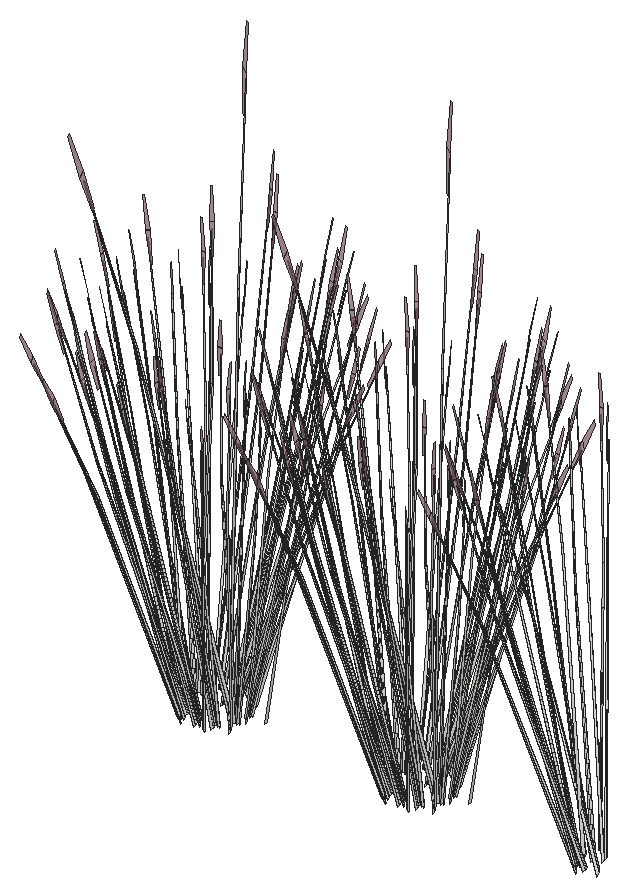
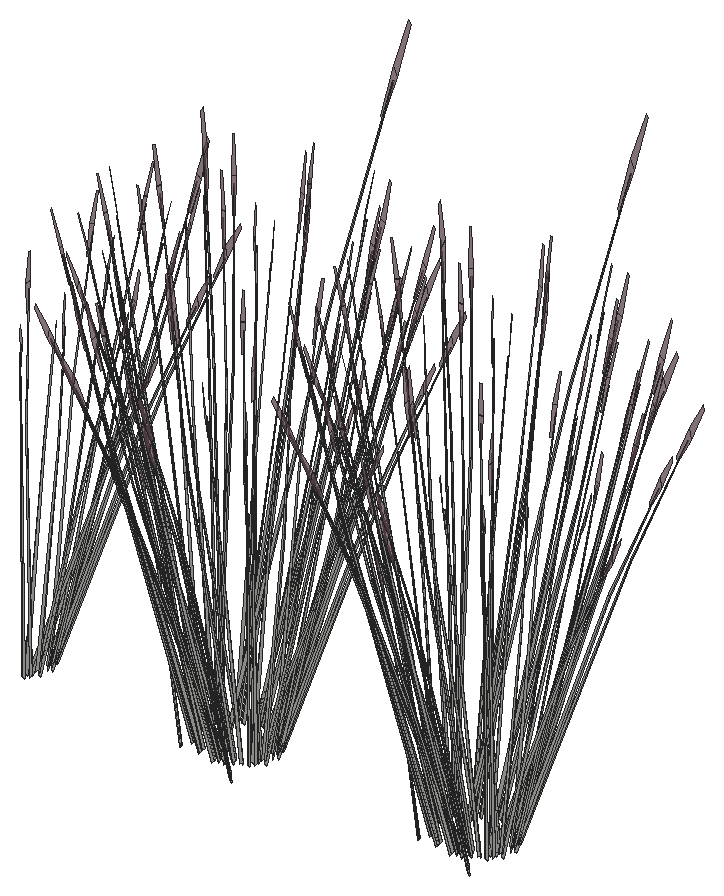
# SketchUp Ruby script. Lengths in inches.
U = 1.inch
M = Sketchup.active_model
def pt(a) = Geom::Point3d.new(a.map { |v| v * U })
def face(e, loops, mat)
  f = e.add_face(loops[0].map { |a| pt(a) })
  loops[1..].each { |l| e.add_face(l.map { |a| pt(a) }).erase! }
  f.material = f.back_material = mat if mat
  f
end
# faces: each face lists its corners as indices into pts; further lists are holes
def faces(e, pts, list, mat = nil) = list.each { |f| face(e, (f[0].is_a?(Array) ? f : [f]).map { |l| l.map { |i| pts[i] } }, mat) }
# xy, xz, yz: faces in a plane at the given z, y or x. An outline is a flat list of corners, or four numbers for a rectangle; further outlines are holes
def ring(l) = l.size == 4 ? [[l[0], l[1]], [l[2], l[1]], [l[2], l[3]], [l[0], l[3]]] : l.each_slice(2).to_a
def flat(e, list, mat, &to3) = list.each { |f| face(e, (f[0].is_a?(Array) ? f : [f]).map { |l| ring(l).map { |u, v| to3.(u, v) } }, mat) }
def xy(e, z, list, mat = nil) = flat(e, list, mat) { |x, y| [x, y, z] }
def xz(e, y, list, mat = nil) = flat(e, list, mat) { |x, z| [x, y, z] }
def yz(e, x, list, mat = nil) = flat(e, list, mat) { |y, z| [x, y, z] }
def lines(e, pts, list) = list.each { |a, b| e.add_line(pt(pts[a]), pt(pts[b])) }
# prism: a flat outline (further loops are holes) pulled along v
def prism(e, loops, v, mat = nil)
  f = face(e, loops, mat); d = Geom::Vector3d.new(v.map { |x| x * U })
  f.pushpull(f.normal.samedirection?(d) ? d.length : -d.length)
end
def box(e, o, s, mat = nil) = prism(e, [[o, [o[0] + s[0], o[1], o[2]], [o[0] + s[0], o[1] + s[1], o[2]], [o[0], o[1] + s[1], o[2]]]], [0, 0, s[2]], mat)
def at(x, y, z, deg = 0) = Geom::Transformation.translation(pt([x, y, z])) * Geom::Transformation.rotation(ORIGIN, Z_AXIS, deg.degrees)
def axes(o, x, y, z) = Geom::Transformation.new([*x, 0, *y, 0, *z, 0, *pt(o).to_a, 1])
def part(name) = M.definitions.add(name)
# library, detail: a bought-in or finely detailed component or shape, given as its bounding box
def library(name, o, s) = part(name).tap { |d| box(d.entities, o, s) }
def detail(e, o, s) = box(e.add_group.entities, o, s)
def put(e, d, t, mat = nil) = e.add_instance(d, t).tap { |i| i.material = mat if mat }
def group(e, t, mat = nil) = e.add_group.tap { |g| g.transformation = t; g.material = mat if mat }.entities
root = M.entities
M.materials.add("LightPink_Translucent").color = [144, 107, 117]
M.materials["LightPink_Translucent"].alpha = 0.75
c1 = part("blade")
p = [[2.15,0.21,22],[0,0.17,0],[0.09,0.45,0],[2.18,0.31,22],[2.29,0.31,22],[0.38,0.45,0],
  [2.48,0.24,33],[2.49,0.24,33],[2.48,0.22,33]]
faces(c1.entities,p,[[0,1,2,3],[4,5,2,3],[6,3,4,7],[8,0,3,6]])
c2 = part("seeds")
p = [[0.3,-0.1,1.38],[-0.01,-0.03,1.59],[-0.01,-0.03,0.03],[0.14,-0.07,-0.07],[0.29,-0.03,3],[0.15,0.01,3.11]]
faces(c2.entities,p,[[0,1,2,3],[1,0,4,5]],"LightPink_Translucent")
c3 = part("blade with seeds")
put(c3.entities,c1,at(0,0,0))
put(c3.entities,c2,axes([2.4,0.25,30.99],[1.5799,-0.05474,1.17369],[-0.12525,1.92788,0.29478],[-0.07173,-0.02425,1.56792]))
put(root,c3,axes([283.23,56.33,267.61],[0.21212,-0.01231,1.59586],[-0.14072,0.53355,0.12904],[-0.3023,-0.033,0.68222]))
put(root,c3,axes([283.32,57.27,267.61],[0.17745,-0.11497,1.59586],[0.14939,0.53127,0.12904],[-0.27857,0.12007,0.68222]))
put(root,c3,axes([284.33,56.71,267.11],[0.14537,-0.07863,1.64882],[0.05013,0.549,0.12904],[-0.31487,0.07285,0.5893]))
put(root,c3,axes([283.86,55.83,268.64],[-0.51122,-0.01309,-0.66157],[0.03434,-0.5511,0.07984],[-0.21658,-0.05816,0.93586]))
put(root,c3,axes([283.04,56.79,268.22],[-0.42502,-0.15163,-0.32977],[0.12396,-0.44238,0.42575],[-0.17112,0.04056,0.81462]))
put(root,c3,axes([283.63,55.47,267.61],[0.18996,0.09365,1.59586],[-0.39312,0.39287,0.12904],[-0.24502,-0.17723,0.68222]))
put(root,c3,axes([283.33,57.01,268.36],[-0.13855,0.49442,-0.47583],[-0.47502,-0.16947,-0.36857],[-0.19125,0.04534,0.91046]))
put(root,c3,axes([283.69,55.94,268.36],[-0.37135,0.36005,-0.47583],[-0.32522,-0.38035,-0.36857],[-0.18868,-0.05478,0.91046]))
put(root,c3,axes([283.31,56.59,268.6875],[0.25732,0.49218,-0.11324],[-0.45669,0.24187,-0.62851],[-0.19245,0.06494,0.95501]))
put(root,c3,axes([283.89,55.57,268.6875],[-0.02738,0.55277,-0.11324],[-0.51847,-0.01511,-0.62851],[-0.19968,-0.0384,0.95501]))
put(root,c3,axes([283.55,55.6,268.22],[-0.29098,-0.34031,-0.32977],[0.33226,-0.32215,0.42575],[-0.16881,-0.04902,0.81462]))
put(root,c3,axes([283.96,57.625,267.61],[0.12773,-0.16701,1.59586],[0.32252,0.4508,0.12904],[-0.22121,0.20529,0.68222]))
put(root,c3,axes([283.2,58.0625,268.22],[-0.44516,0.07768,-0.32977],[-0.11755,-0.44407,0.42575],[-0.12757,0.11927,0.81462]))
put(root,c3,axes([283.87,58.04,267.61],[0.09522,-0.18683,1.59586],[0.39947,0.38663,0.12904],[-0.18021,0.24097,0.68222]))
put(root,c3,axes([283.5625,58.11,268.36],[0.13138,0.49631,-0.47583],[-0.49754,0.08682,-0.36857],[-0.14258,0.13331,0.91046]))
put(root,c3,axes([284.75,55.18,268.64],[-0.43608,-0.26272,-0.66157],[0.30991,-0.46038,0.07984],[-0.158,-0.15687,0.93586]))
put(root,c3,axes([284.55,55.2,268.36],[-0.50465,0.12921,-0.47583],[-0.08828,-0.48932,-0.36857],[-0.13555,-0.14022,0.91046]))
put(root,c3,axes([283.33,57.76,268.6875],[0.47307,0.29971,-0.11324],[-0.27254,0.43404,-0.62851],[-0.13365,0.15087,0.95501]))
put(root,c3,axes([284.41,54.93,267.61],[0.1169,0.17452,1.59586],[-0.54019,0.14692,0.12904],[-0.12209,-0.27397,0.68222]))
put(root,c3,axes([284.6,54.83,268.22],[-0.07899,-0.43781,-0.32977],[0.45153,-0.11561,0.42575],[-0.12128,-0.12546,0.81462]))
put(root,c3,axes([283.98,59.09,268.22],[-0.34603,0.28618,-0.32977],[-0.32756,-0.32677,0.42575],[-0.04984,0.16603,0.81462]))
put(root,c3,axes([285.79,58.15,267.1],[0.44194,0.21918,1.40854],[-0.43295,0.47219,0.557],[-0.19393,-0.27986,1.18082]))
put(root,c3,axes([284.21,58.79,268.97],[-0.01331,0.50278,-0.73435],[-0.56035,-0.03377,0.08862],[-0.05914,0.213,1.03881]))
put(root,c3,axes([284.02,59.5,267.13],[0.01124,-0.2806,1.43727],[0.50537,0.14821,0.19862],[-0.04379,0.29905,0.67868]))
put(root,c3,axes([284.32,58.95,268.66],[0.3661,0.36521,-0.52818],[-0.38674,0.31985,-0.40911],[-0.0557,0.18556,1.01061]))
put(root,c3,axes([286.48,57.11,266.65],[-0.01397,-0.51177,1.31553],[0.63227,0.13266,0.557],[-0.14954,0.28003,1.24175]))
put(root,c3,axes([286.1,54.95,268.6875],[-0.50045,0.25306,-0.11324],[-0.24593,-0.44915,-0.62851],[-0.06603,-0.18927,0.95501]))
put(root,c3,axes([285.67,54.97,268.36],[-0.50273,-0.13626,-0.47583],[0.17232,-0.46717,-0.36857],[-0.0461,-0.18809,0.91046]))
put(root,c3,axes([284.74,58.43,267.61],[-0.01252,-0.20862,1.59586],[0.54251,0.1384,0.12904],[-0.03356,0.2973,0.68222]))
put(root,c3,axes([285.85,55.06,268.64],[-0.24409,-0.44196,-0.66157],[0.50245,-0.2463,0.07984],[-0.05708,-0.21354,0.93586]))
put(root,c3,axes([285.9,54.68,268.22],[0.15418,-0.41799,-0.32977],[0.44981,0.12192,0.42575],[-0.04124,-0.16829,0.81462]))
put(root,c3,axes([285.18,59.59,268.22],[-0.15418,0.41799,-0.32977],[-0.44981,-0.12192,0.42575],[0.04124,0.16829,0.81462]))
put(root,c3,axes([285.23,59.22,268.64],[0.24409,0.44196,-0.66157],[-0.50245,0.2463,0.07984],[0.05708,0.21354,0.93586]))
put(root,c3,axes([285.41,59.31,268.36],[0.50273,0.13626,-0.47583],[-0.17232,0.46717,-0.36857],[0.0461,0.18809,0.91046]))
put(root,c3,axes([284.98,59.33,268.6875],[0.50045,-0.25306,-0.11324],[0.24593,0.44915,-0.62851],[0.06603,0.18927,0.95501]))
put(root,c3,axes([287.14,55.51,268.6875],[-0.56206,-0.02693,-0.11324],[0.01536,-0.50991,-0.62851],[0.03904,-0.19638,0.95501]))
put(root,c3,axes([286.75,55.32,268.36],[-0.3661,-0.36521,-0.47583],[0.38674,-0.31985,-0.36857],[0.0557,-0.18556,0.91046]))
put(root,c3,axes([285.69,58.34,267.61],[-0.1169,-0.17452,1.59586],[0.54019,-0.14692,0.12904],[0.12209,0.27397,0.68222]))
put(root,c3,axes([286.87,55.49,268.64],[0.01331,-0.50278,-0.66157],[0.56035,0.03377,0.07984],[0.05914,-0.213,0.93586]))
put(root,c3,axes([287.1,55.1875,268.22],[0.34603,-0.28618,-0.32977],[0.32756,0.32677,0.42575],[0.04984,-0.16603,0.81462]))
put(root,c3,axes([286.24,55.23,267.61],[-0.09522,0.18683,1.59586],[-0.39947,-0.38663,0.12904],[0.18021,-0.24097,0.68222]))
put(root,c3,axes([286.17,59.3125,268.6875],[0.30474,-0.46525,-0.11324],[0.44133,0.26804,-0.62851],[0.15341,0.13145,0.95501]))
put(root,c3,axes([287.75,56.52,268.6875],[-0.47307,-0.29971,-0.11324],[0.27254,-0.43404,-0.62851],[0.13365,-0.15087,0.95501]))
put(root,c3,axes([286.53,59.08,268.36],[0.50465,-0.12921,-0.47583],[0.08828,0.48932,-0.36857],[0.13555,0.14022,0.91046]))
put(root,c3,axes([287.51,56.16,268.36],[-0.13138,-0.49631,-0.47583],[0.49754,-0.08682,-0.36857],[0.14258,-0.13331,0.91046]))
put(root,c3,axes([288.39,58.72,267.66],[-0.09788,-0.45691,-0.03251],[0.46264,-0.10504,-0.14742],[0.09661,0.02897,0.48626]))
put(root,c3,axes([286.48,57.8,267.61],[-0.18996,-0.09365,1.59586],[0.39312,-0.39287,0.12904],[0.24502,0.17723,0.68222]))
put(root,c3,axes([287.88,56.22,268.22],[0.44516,-0.07768,-0.32977],[0.11755,0.44407,0.42575],[0.12757,-0.11927,0.81462]))
put(root,c3,axes([287.53,56.36,268.64],[0.26714,-0.42887,-0.66157],[0.46811,0.30479,0.07984],[0.1595,-0.15539,0.93586]))
put(root,c3,axes([287.52,58.67,268.22],[0.29098,0.34031,-0.32977],[-0.33226,0.32215,0.42575],[0.16881,0.04902,0.81462]))
put(root,c3,axes([287.1875,58.71,268.6875],[0.02738,-0.55277,-0.11324],[0.51847,0.01511,-0.62851],[0.19968,0.0384,0.95501]))
put(root,c3,axes([287.77,57.6875,268.6875],[-0.25732,-0.49218,-0.11324],[0.45669,-0.24187,-0.62851],[0.19245,-0.06494,0.95501]))
put(root,c3,axes([287.74,57.27,268.36],[0.13855,-0.49442,-0.47583],[0.47502,0.16947,-0.36857],[0.19125,-0.04534,0.91046]))
put(root,c3,axes([288.04,57.49,268.22],[0.42502,0.15163,-0.32977],[-0.12396,0.44238,0.42575],[0.17112,-0.04056,0.81462]))
put(root,c3,axes([287.21,58.44,268.64],[0.51122,0.01309,-0.66157],[-0.03434,0.5511,0.07984],[0.21658,0.05816,0.93586]))
put(root,c3,axes([286.88,56.94,267.61],[-0.21212,0.01231,1.59586],[0.14072,-0.53355,0.12904],[0.3023,0.033,0.68222]))
put(root,c3,axes([287.65,57.45,268.64],[0.44939,-0.24006,-0.66157],[0.25044,0.49415,0.07984],[0.21713,-0.05613,0.93586]))
put(root,c3,axes([300.45,56.33,267.61],[0.21212,-0.01231,1.59586],[-0.14072,0.53355,0.12904],[-0.3023,-0.033,0.68222]))
put(root,c3,axes([300.53,57.27,267.61],[0.17745,-0.11497,1.59586],[0.14939,0.53127,0.12904],[-0.27857,0.12007,0.68222]))
put(root,c3,axes([301.55,56.71,267.11],[0.14537,-0.07863,1.64882],[0.05013,0.549,0.12904],[-0.31487,0.07285,0.5893]))
put(root,c3,axes([301.08,55.83,268.64],[-0.51122,-0.01309,-0.66157],[0.03434,-0.5511,0.07984],[-0.21658,-0.05816,0.93586]))
put(root,c3,axes([300.26,56.79,268.22],[-0.42502,-0.15163,-0.32977],[0.12396,-0.44238,0.42575],[-0.17112,0.04056,0.81462]))
put(root,c3,axes([300.85,55.47,267.61],[0.18996,0.09365,1.59586],[-0.39312,0.39287,0.12904],[-0.24502,-0.17723,0.68222]))
put(root,c3,axes([300.55,57.01,268.36],[-0.13855,0.49442,-0.47583],[-0.47502,-0.16947,-0.36857],[-0.19125,0.04534,0.91046]))
put(root,c3,axes([300.91,55.94,268.36],[-0.37135,0.36005,-0.47583],[-0.32522,-0.38035,-0.36857],[-0.18868,-0.05478,0.91046]))
put(root,c3,axes([300.53,56.59,268.6875],[0.25732,0.49218,-0.11324],[-0.45669,0.24187,-0.62851],[-0.19245,0.06494,0.95501]))
put(root,c3,axes([301.11,55.57,268.6875],[-0.02738,0.55277,-0.11324],[-0.51847,-0.01511,-0.62851],[-0.19968,-0.0384,0.95501]))
put(root,c3,axes([300.77,55.6,268.22],[-0.29098,-0.34031,-0.32977],[0.33226,-0.32215,0.42575],[-0.16881,-0.04902,0.81462]))
put(root,c3,axes([301.18,57.625,267.61],[0.12773,-0.16701,1.59586],[0.32252,0.4508,0.12904],[-0.22121,0.20529,0.68222]))
put(root,c3,axes([300.42,58.0625,268.22],[-0.44516,0.07768,-0.32977],[-0.11755,-0.44407,0.42575],[-0.12757,0.11927,0.81462]))
put(root,c3,axes([301.09,58.04,267.61],[0.09522,-0.18683,1.59586],[0.39947,0.38663,0.12904],[-0.18021,0.24097,0.68222]))
put(root,c3,axes([300.78,58.11,268.36],[0.13138,0.49631,-0.47583],[-0.49754,0.08682,-0.36857],[-0.14258,0.13331,0.91046]))
put(root,c3,axes([301.97,55.18,268.64],[-0.43608,-0.26272,-0.66157],[0.30991,-0.46038,0.07984],[-0.158,-0.15687,0.93586]))
put(root,c3,axes([301.77,55.2,268.36],[-0.50465,0.12921,-0.47583],[-0.08828,-0.48932,-0.36857],[-0.13555,-0.14022,0.91046]))
put(root,c3,axes([300.55,57.76,268.6875],[0.47307,0.29971,-0.11324],[-0.27254,0.43404,-0.62851],[-0.13365,0.15087,0.95501]))
put(root,c3,axes([301.63,54.93,267.61],[0.1169,0.17452,1.59586],[-0.54019,0.14692,0.12904],[-0.12209,-0.27397,0.68222]))
put(root,c3,axes([301.82,54.83,268.22],[-0.07899,-0.43781,-0.32977],[0.45153,-0.11561,0.42575],[-0.12128,-0.12546,0.81462]))
put(root,c3,axes([301.2,59.09,268.22],[-0.34603,0.28618,-0.32977],[-0.32756,-0.32677,0.42575],[-0.04984,0.16603,0.81462]))
put(root,c3,axes([303.01,58.15,267.1],[0.44194,0.21918,1.40854],[-0.43295,0.47219,0.557],[-0.19393,-0.27986,1.18082]))
put(root,c3,axes([301.43,58.79,268.97],[-0.01331,0.50278,-0.73435],[-0.56035,-0.03377,0.08862],[-0.05914,0.213,1.03881]))
put(root,c3,axes([301.24,59.5,267.13],[0.01124,-0.2806,1.43727],[0.50537,0.14821,0.19862],[-0.04379,0.29905,0.67868]))
put(root,c3,axes([301.54,58.95,268.66],[0.3661,0.36521,-0.52818],[-0.38674,0.31985,-0.40911],[-0.0557,0.18556,1.01061]))
put(root,c3,axes([303.7,57.11,266.65],[-0.01397,-0.51177,1.31553],[0.63227,0.13266,0.557],[-0.14954,0.28003,1.24175]))
put(root,c3,axes([303.32,54.95,268.6875],[-0.50045,0.25306,-0.11324],[-0.24593,-0.44915,-0.62851],[-0.06603,-0.18927,0.95501]))
put(root,c3,axes([302.89,54.97,268.36],[-0.50273,-0.13626,-0.47583],[0.17232,-0.46717,-0.36857],[-0.0461,-0.18809,0.91046]))
put(root,c3,axes([301.96,58.43,267.61],[-0.01252,-0.20862,1.59586],[0.54251,0.1384,0.12904],[-0.03356,0.2973,0.68222]))
put(root,c3,axes([303.07,55.06,268.64],[-0.24409,-0.44196,-0.66157],[0.50245,-0.2463,0.07984],[-0.05708,-0.21354,0.93586]))
put(root,c3,axes([303.12,54.68,268.22],[0.15418,-0.41799,-0.32977],[0.44981,0.12192,0.42575],[-0.04124,-0.16829,0.81462]))
put(root,c3,axes([302.4,59.59,268.22],[-0.15418,0.41799,-0.32977],[-0.44981,-0.12192,0.42575],[0.04124,0.16829,0.81462]))
put(root,c3,axes([302.45,59.22,268.64],[0.24409,0.44196,-0.66157],[-0.50245,0.2463,0.07984],[0.05708,0.21354,0.93586]))
put(root,c3,axes([302.63,59.31,268.36],[0.50273,0.13626,-0.47583],[-0.17232,0.46717,-0.36857],[0.0461,0.18809,0.91046]))
put(root,c3,axes([302.2,59.33,268.6875],[0.50045,-0.25306,-0.11324],[0.24593,0.44915,-0.62851],[0.06603,0.18927,0.95501]))
put(root,c3,axes([304.36,55.51,268.6875],[-0.56206,-0.02693,-0.11324],[0.01536,-0.50991,-0.62851],[0.03904,-0.19638,0.95501]))
put(root,c3,axes([303.97,55.32,268.36],[-0.3661,-0.36521,-0.47583],[0.38674,-0.31985,-0.36857],[0.0557,-0.18556,0.91046]))
put(root,c3,axes([302.91,58.34,267.61],[-0.1169,-0.17452,1.59586],[0.54019,-0.14692,0.12904],[0.12209,0.27397,0.68222]))
put(root,c3,axes([304.09,55.49,268.64],[0.01331,-0.50278,-0.66157],[0.56035,0.03377,0.07984],[0.05914,-0.213,0.93586]))
put(root,c3,axes([304.32,55.1875,268.22],[0.34603,-0.28618,-0.32977],[0.32756,0.32677,0.42575],[0.04984,-0.16603,0.81462]))
put(root,c3,axes([303.46,55.23,267.61],[-0.09522,0.18683,1.59586],[-0.39947,-0.38663,0.12904],[0.18021,-0.24097,0.68222]))
put(root,c3,axes([303.39,59.3125,268.6875],[0.30474,-0.46525,-0.11324],[0.44133,0.26804,-0.62851],[0.15341,0.13145,0.95501]))
put(root,c3,axes([304.97,56.52,268.6875],[-0.47307,-0.29971,-0.11324],[0.27254,-0.43404,-0.62851],[0.13365,-0.15087,0.95501]))
put(root,c3,axes([303.75,59.08,268.36],[0.50465,-0.12921,-0.47583],[0.08828,0.48932,-0.36857],[0.13555,0.14022,0.91046]))
put(root,c3,axes([304.73,56.16,268.36],[-0.13138,-0.49631,-0.47583],[0.49754,-0.08682,-0.36857],[0.14258,-0.13331,0.91046]))
put(root,c3,axes([305.61,58.72,267.66],[-0.09788,-0.45691,-0.03251],[0.46264,-0.10504,-0.14742],[0.09661,0.02897,0.48626]))
put(root,c3,axes([303.7,57.8,267.61],[-0.18996,-0.09365,1.59586],[0.39312,-0.39287,0.12904],[0.24502,0.17723,0.68222]))
put(root,c3,axes([305.1,56.22,268.22],[0.44516,-0.07768,-0.32977],[0.11755,0.44407,0.42575],[0.12757,-0.11927,0.81462]))
put(root,c3,axes([304.75,56.36,268.64],[0.26714,-0.42887,-0.66157],[0.46811,0.30479,0.07984],[0.1595,-0.15539,0.93586]))
put(root,c3,axes([304.74,58.67,268.22],[0.29098,0.34031,-0.32977],[-0.33226,0.32215,0.42575],[0.16881,0.04902,0.81462]))
put(root,c3,axes([304.41,58.71,268.6875],[0.02738,-0.55277,-0.11324],[0.51847,0.01511,-0.62851],[0.19968,0.0384,0.95501]))
put(root,c3,axes([304.99,57.6875,268.6875],[-0.25732,-0.49218,-0.11324],[0.45669,-0.24187,-0.62851],[0.19245,-0.06494,0.95501]))
put(root,c3,axes([304.96,57.26,268.36],[0.13855,-0.49442,-0.47583],[0.47502,0.16947,-0.36857],[0.19125,-0.04534,0.91046]))
put(root,c3,axes([305.26,57.49,268.22],[0.42502,0.15163,-0.32977],[-0.12396,0.44238,0.42575],[0.17112,-0.04056,0.81462]))
put(root,c3,axes([304.43,58.44,268.64],[0.51122,0.01309,-0.66157],[-0.03434,0.5511,0.07984],[0.21658,0.05816,0.93586]))
put(root,c3,axes([304.1,56.94,267.61],[-0.21212,0.01231,1.59586],[0.14072,-0.53355,0.12904],[0.3023,0.033,0.68222]))
put(root,c3,axes([304.875,57.45,268.64],[0.44939,-0.24006,-0.66157],[0.25044,0.49415,0.07984],[0.21713,-0.05613,0.93586]))
put(root,c3,axes([316.81,56.33,267.61],[0.21212,-0.01231,1.59586],[-0.14072,0.53355,0.12904],[-0.3023,-0.033,0.68222]))
put(root,c3,axes([316.9,57.27,267.61],[0.17745,-0.11497,1.59586],[0.14939,0.53127,0.12904],[-0.27857,0.12007,0.68222]))
put(root,c3,axes([317.92,56.71,267.11],[0.14537,-0.07863,1.64882],[0.05013,0.549,0.12904],[-0.31487,0.07285,0.5893]))
put(root,c3,axes([317.44,55.83,268.64],[-0.51122,-0.01309,-0.66157],[0.03434,-0.5511,0.07984],[-0.21658,-0.05816,0.93586]))
put(root,c3,axes([316.62,56.79,268.22],[-0.42502,-0.15163,-0.32977],[0.12396,-0.44238,0.42575],[-0.17112,0.04056,0.81462]))
put(root,c3,axes([317.21,55.47,267.61],[0.18996,0.09365,1.59586],[-0.39312,0.39287,0.12904],[-0.24502,-0.17723,0.68222]))
put(root,c3,axes([316.91,57.01,268.36],[-0.13855,0.49442,-0.47583],[-0.47502,-0.16947,-0.36857],[-0.19125,0.04534,0.91046]))
put(root,c3,axes([317.27,55.94,268.36],[-0.37135,0.36005,-0.47583],[-0.32522,-0.38035,-0.36857],[-0.18868,-0.05478,0.91046]))
put(root,c3,axes([316.89,56.59,268.6875],[0.25732,0.49218,-0.11324],[-0.45669,0.24187,-0.62851],[-0.19245,0.06494,0.95501]))
put(root,c3,axes([317.47,55.57,268.6875],[-0.02738,0.55277,-0.11324],[-0.51847,-0.01511,-0.62851],[-0.19968,-0.0384,0.95501]))
put(root,c3,axes([317.14,55.6,268.22],[-0.29098,-0.34031,-0.32977],[0.33226,-0.32215,0.42575],[-0.16881,-0.04902,0.81462]))
put(root,c3,axes([317.55,57.625,267.61],[0.12773,-0.16701,1.59586],[0.32252,0.4508,0.12904],[-0.22121,0.20529,0.68222]))
put(root,c3,axes([316.78,58.0625,268.22],[-0.44516,0.07768,-0.32977],[-0.11755,-0.44407,0.42575],[-0.12757,0.11927,0.81462]))
put(root,c3,axes([317.45,58.04,267.61],[0.09522,-0.18683,1.59586],[0.39947,0.38663,0.12904],[-0.18021,0.24097,0.68222]))
put(root,c3,axes([317.15,58.11,268.36],[0.13138,0.49631,-0.47583],[-0.49754,0.08682,-0.36857],[-0.14258,0.13331,0.91046]))
put(root,c3,axes([318.33,55.18,268.64],[-0.43608,-0.26272,-0.66157],[0.30991,-0.46038,0.07984],[-0.158,-0.15687,0.93586]))
